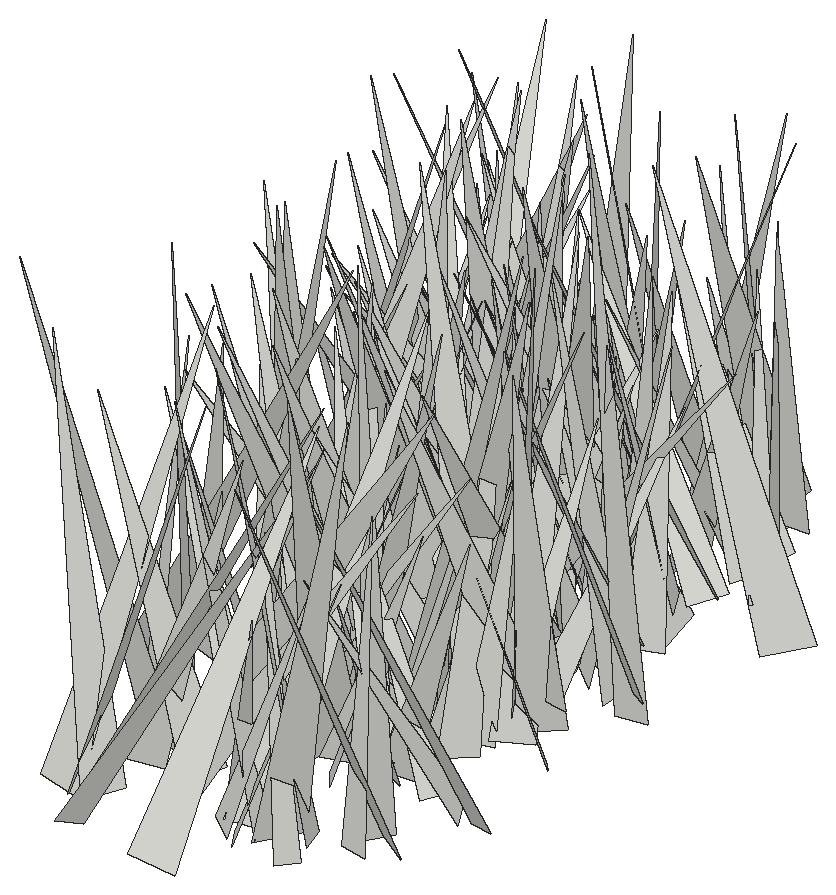
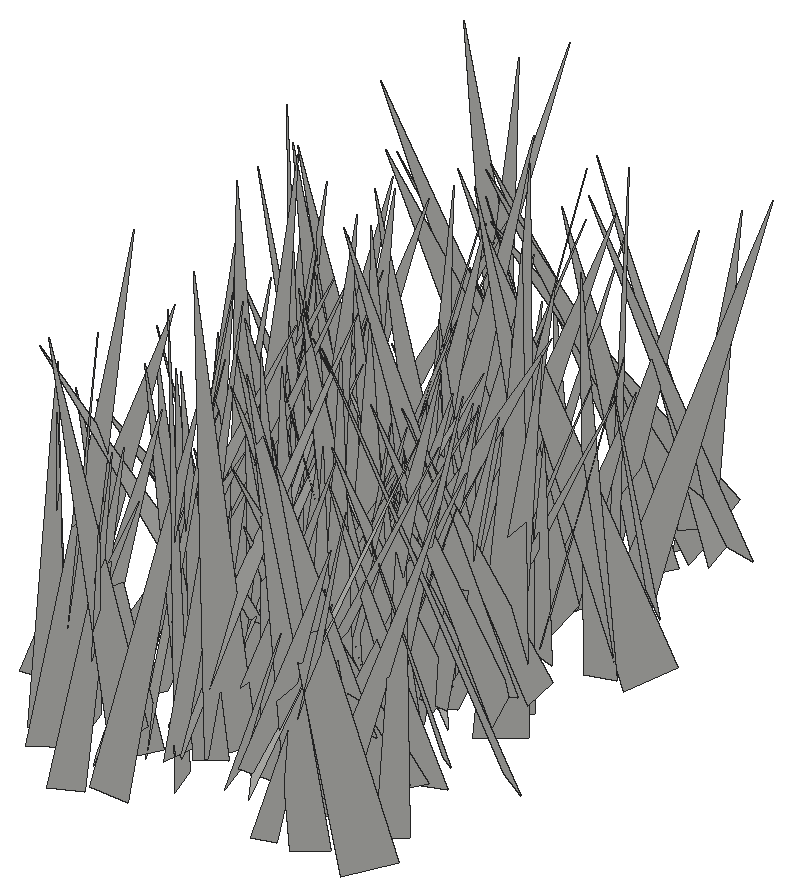
# SketchUp Ruby script. Lengths in inches.
U = 1.inch
M = Sketchup.active_model
def pt(a) = Geom::Point3d.new(a.map { |v| v * U })
def face(e, loops, mat)
  f = e.add_face(loops[0].map { |a| pt(a) })
  loops[1..].each { |l| e.add_face(l.map { |a| pt(a) }).erase! }
  f.material = f.back_material = mat if mat
  f
end
# faces: each face lists its corners as indices into pts; further lists are holes
def faces(e, pts, list, mat = nil) = list.each { |f| face(e, (f[0].is_a?(Array) ? f : [f]).map { |l| l.map { |i| pts[i] } }, mat) }
# xy, xz, yz: faces in a plane at the given z, y or x. An outline is a flat list of corners, or four numbers for a rectangle; further outlines are holes
def ring(l) = l.size == 4 ? [[l[0], l[1]], [l[2], l[1]], [l[2], l[3]], [l[0], l[3]]] : l.each_slice(2).to_a
def flat(e, list, mat, &to3) = list.each { |f| face(e, (f[0].is_a?(Array) ? f : [f]).map { |l| ring(l).map { |u, v| to3.(u, v) } }, mat) }
def xy(e, z, list, mat = nil) = flat(e, list, mat) { |x, y| [x, y, z] }
def xz(e, y, list, mat = nil) = flat(e, list, mat) { |x, z| [x, y, z] }
def yz(e, x, list, mat = nil) = flat(e, list, mat) { |y, z| [x, y, z] }
def lines(e, pts, list) = list.each { |a, b| e.add_line(pt(pts[a]), pt(pts[b])) }
# prism: a flat outline (further loops are holes) pulled along v
def prism(e, loops, v, mat = nil)
  f = face(e, loops, mat); d = Geom::Vector3d.new(v.map { |x| x * U })
  f.pushpull(f.normal.samedirection?(d) ? d.length : -d.length)
end
def box(e, o, s, mat = nil) = prism(e, [[o, [o[0] + s[0], o[1], o[2]], [o[0] + s[0], o[1] + s[1], o[2]], [o[0], o[1] + s[1], o[2]]]], [0, 0, s[2]], mat)
def at(x, y, z, deg = 0) = Geom::Transformation.translation(pt([x, y, z])) * Geom::Transformation.rotation(ORIGIN, Z_AXIS, deg.degrees)
def axes(o, x, y, z) = Geom::Transformation.new([*x, 0, *y, 0, *z, 0, *pt(o).to_a, 1])
def part(name) = M.definitions.add(name)
# library, detail: a bought-in or finely detailed component or shape, given as its bounding box
def library(name, o, s) = part(name).tap { |d| box(d.entities, o, s) }
def detail(e, o, s) = box(e.add_group.entities, o, s)
def put(e, d, t, mat = nil) = e.add_instance(d, t).tap { |i| i.material = mat if mat }
def group(e, t, mat = nil) = e.add_group.tap { |g| g.transformation = t; g.material = mat if mat }.entities
root = M.entities
c1 = part("fur_instance\#9")
p = [[0.8125,0,1.79],[0.67,-0.02,1.48],[0,-0.11,0],[0,0.11,0]]
faces(c1.entities,p,[[0,1,2,3]])
put(root,c1,axes([89.89,190.3,-27.1],[-4.18916,1.41328,1.44955],[1.84035,4.04661,1.3732],[0.84361,-1.80976,4.20247]))
put(root,c1,axes([88.07,187.8,-27.1],[2.28219,3.09258,0.57784],[3.14608,-2.24088,-0.43237],[0.01087,-0.72161,3.81909]))
put(root,c1,axes([86.96,186.11,-28.22],[4.54632,6.46757,0.61256],[6.48609,-4.47646,-0.87508],[0.36794,-1.0028,7.85702]))
put(root,c1,axes([91.4,174.74,-28.22],[-2.64388,-6.79077,2.11498],[-6.99476,2.07362,-2.08599],[-1.28885,2.67645,6.98236]))
put(root,c1,axes([87.72,190.74,-28.22],[5.48383,-1.63022,0.30334],[-1.45467,-5.23263,-1.82362],[-0.79597,-1.66854,5.42259]))
put(root,c1,axes([88.75,184.4,-27.1],[5.94248,2.0649,1.47313],[1.51819,-5.90154,2.14801],[-2.032,1.62942,5.91295]))
put(root,c1,axes([90.75,181.75,-27.1],[-5.69821,2.17721,0.97614],[2.15034,5.78116,-0.34192],[1.034,-0.02439,6.0904]))
put(root,c1,axes([90.47,175.18,-28.22],[2.37609,4.94692,0.8109],[4.47755,-2.49789,2.11838],[-2.25414,0.25283,5.06264]))
put(root,c1,axes([91.61,192.51,-27.1],[-5.39414,-3.77764,0.22745],[-3.78403,5.38986,-0.22257],[0.05845,0.31282,6.58162]))
put(root,c1,axes([90.58,188.05,-28.22],[-6.26748,-0.84521,1.62615],[-0.68504,6.45447,0.7145],[1.69984,-0.51518,6.28372]))
put(root,c1,axes([91.5625,190.9,-28.22],[-6.30755,-1.0303,0.95825],[-1.23667,6.15876,-1.51833],[0.67114,1.66527,6.20817]))
put(root,c1,axes([88.71,187.71,-28.22],[0.12132,5.40428,1.16344],[5.42728,0.10479,-1.05269],[1.05091,-1.16504,5.30215]))
put(root,c1,axes([89.95,191.67,-27.1],[4.40481,-2.70951,0.82389],[-1.71706,-3.76665,-3.20728],[-2.2521,-2.42766,4.05674]))
put(root,c1,axes([90.42,189.11,-27.1],[-4.33285,5.33033,0.39838],[5.19442,4.31986,-1.30443],[1.26061,0.52067,6.74422]))
put(root,c1,axes([89.58,190.12,-28.22],[1.06055,3.50039,1.15885],[3.68372,-1.05849,-0.17402],[-0.16095,-1.16074,3.65339]))
put(root,c1,axes([88.96,184.14,-28.22],[5.45655,-4.97036,1.37233],[-4.9464,-5.60993,-0.6508],[-1.45634,0.43117,7.35221]))
put(root,c1,axes([91.19,179.65,-28.22],[-0.14147,5.00237,0.6936],[4.87308,-0.04695,1.33257],[-1.32587,-0.70632,4.82369]))
put(root,c1,axes([91.25,183.76,-28.22],[-5.28354,-0.86585,0.73138],[-0.45173,4.80676,2.42722],[1.0395,-2.31209,4.77222]))
put(root,c1,axes([91.92,187.52,-28.22],[-1.59145,-6.67923,2.98055],[-7.18236,0.85085,-1.92829],[-1.38185,3.26993,6.58988]))
put(root,c1,axes([88.44,182.95,-27.1],[5.14686,-0.10254,0.48257],[-0.21946,-5.00543,1.27711],[-0.44184,1.29176,4.98695]))
put(root,c1,axes([88.93,179.57,-28.22],[-0.17668,-5.97479,1.5156],[-5.97573,0.53792,1.42395],[1.51188,1.4279,5.80532]))
put(root,c1,axes([92.4,190,-27.1],[-5.87087,-0.65311,0.1721],[-0.62527,5.82501,0.77566],[0.25536,-0.75237,5.85594]))
put(root,c1,axes([91.77,171.64,-28.22],[-6.40273,2.01611,1.14645],[1.98655,6.50456,-0.34415],[1.19695,-0.01086,6.70383]))
put(root,c1,axes([90.48,185.39,-27.1],[-0.08561,-4.51883,0.61864],[-4.55746,0.06047,-0.18896],[-0.17898,0.62161,4.51569]))
put(root,c1,axes([90.54,193.22,-28.22],[2.63547,-2.52355,0.88422],[-2.24578,-2.7628,-1.19134],[-1.45143,-0.30736,3.44888]))
put(root,c1,axes([91.93,191.88,-27.1],[-2.38269,3.95567,1.05235],[4.03891,2.07425,1.34786],[-0.66484,-1.57548,4.41677]))
put(root,c1,axes([92.6875,180.37,-28.22],[-5.83458,-0.97839,0.23219],[-1.00024,5.78729,-0.74851],[0.10327,0.77686,5.8685]))
put(root,c1,axes([87.0625,192.63,-28.22],[4.73655,-6.32836,0.37656],[-6.13582,-4.45802,2.25891],[1.59428,1.644,7.57499]))
put(root,c1,axes([90.7,176.82,-28.22],[-4.49865,-5.44108,2.87885],[-5.83326,4.90701,0.15896],[1.96626,2.10876,7.05818]))
put(root,c1,axes([92.63,176.8125,-28.22],[-2.13288,4.47426,0.69403],[4.36785,1.83113,1.61826],[-1.19274,-1.2953,4.68502]))
put(root,c1,axes([89.04,183.8125,-27.1],[4.0967,-0.1052,0.02727],[-0.10864,-3.93802,1.12914],[0.00278,1.12946,3.93942]))
put(root,c1,axes([89.52,183.01,-28.22],[7.83218,-2.47016,1.5817],[-2.12062,-7.88445,-1.81244],[-2.02643,-1.29626,8.00998]))
put(root,c1,axes([90.46,182.61,-27.1],[1.50954,-3.07856,1.78204],[-3.55315,-1.39659,0.59714],[-0.16832,1.87187,3.37633]))
put(root,c1,axes([91.59,178.93,-28.22],[-3.92886,-2.51502,0.86647],[-2.44083,4.02285,0.60923],[1.05758,-0.05874,4.62495]))
put(root,c1,axes([91.67,185.23,-28.22],[3.58153,-3.37168,2.12142],[-3.21603,-4.13077,-1.13573],[-2.3507,0.51427,4.78599]))
put(root,c1,axes([92.67,184.25,-27.1],[-3.84784,-1.19504,0.32807],[-1.23606,3.62421,-1.29571],[-0.08892,1.33363,3.81512]))
put(root,c1,axes([90.45,185,-27.1],[4.99403,0.89918,1.35491],[0.3935,-4.91429,1.81096],[-1.5778,1.62046,4.74018]))
put(root,c1,axes([91.96,186.64,-27.1],[-3.17916,-2.57933,0.00353],[-2.53731,3.12837,0.73174],[0.46373,-0.56605,4.02798]))
put(root,c1,axes([89.2,188.12,-28.22],[-0.99691,5.86129,1.26655],[5.41282,1.43213,-2.36709],[2.58075,-0.73958,5.45394]))
put(root,c1,axes([91.16,191.28,-28.22],[5.03177,-2.92165,1.14225],[-2.20313,-4.82824,-2.64459],[-2.23316,-1.81978,5.18275]))
put(root,c1,axes([89.12,192.84,-28.22],[0.83878,-6.84447,1.51714],[-6.71971,-0.34936,2.13903],[1.99848,1.69801,6.55552]))
put(root,c1,axes([89.86,190.82,-28.22],[6.15158,-3.29467,0.71793],[-3.15743,-6.15236,-1.17953],[-1.18361,-0.7112,6.87789]))
put(root,c1,axes([90.54,171.24,-28.22],[1.55056,7.17303,0.47228],[7.18686,-1.53634,-0.26142],[0.15632,-0.51668,7.33405]))
put(root,c1,axes([87.71,178.71,-28.22],[7.56022,-3.29271,0.03526],[-3.23696,-7.41517,1.59297],[0.60437,1.47429,8.09082]))
put(root,c1,axes([92,188.82,-27.1],[-5.13165,1.21269,1.54361],[1.09048,5.35359,-0.58061],[1.63224,0.23592,5.24093]))
put(root,c1,axes([93.08,190.19,-28.22],[-6.30471,-1.37126,0.42808],[-1.05468,5.72683,2.8114],[0.97532,-2.67133,5.80738]))
put(root,c1,axes([89.42,183.91,-27.1],[0.24663,7.62872,2.41582],[7.70784,0.42293,-2.12242],[2.15005,-2.39126,7.33168]))
put(root,c1,axes([93.79,186.91,-28.22],[-0.45254,-7.13046,0.09555],[-6.72101,0.39447,-2.39372],[-2.38342,0.24148,6.7319]))
put(root,c1,axes([89.21,188.96,-28.22],[6.84085,-1.05323,0.60817],[-1.14548,-6.7472,1.19982],[-0.40871,1.28156,6.81667]))
put(root,c1,axes([93.53,190.91,-28.22],[-4.16837,-0.36819,0.02902],[-0.35612,3.91965,-1.4217],[-0.09791,1.41863,3.93569]))
put(root,c1,axes([92.87,181.38,-28.22],[-3.95377,2.90545,0.68572],[2.92437,3.99824,-0.07937],[0.59996,-0.34142,4.90588]))
put(root,c1,axes([93.03,179.86,-28.22],[-4.7653,3.97573,1.88545],[4.327,4.73874,0.94381],[0.79899,-1.95123,6.13381]))
put(root,c1,axes([93.35,174.18,-28.22],[-5.50696,2.25656,1.40845],[2.52369,5.45565,1.12666],[0.84072,-1.59571,5.84374]))
put(root,c1,axes([93.37,184.85,-27.1],[0.69074,-4.72184,2.34998],[-4.89788,-1.45354,-1.48096],[-1.95676,1.97148,4.53648]))
put(root,c1,axes([91.79,177.77,-28.22],[-7.4216,0.05563,3.73189],[-0.80703,8.0859,-1.72548],[3.64401,1.90407,7.21845]))
put(root,c1,axes([93.91,185.04,-28.22],[-6.19983,-0.76734,1.02255],[-1.02443,6.01091,-1.70052],[0.76483,1.83095,6.01123]))
put(root,c1,axes([93.95,190.33,-27.1],[-5.48132,1.03762,0.48302],[1.07413,5.47965,0.41785],[0.39525,-0.50168,5.563]))
put(root,c1,axes([91.5,182.15,-28.22],[5.47744,-1.647,1.93505],[-1.81976,-5.75174,0.25556],[-1.77356,0.81501,5.71398]))
put(root,c1,axes([91.14,187.47,-27.1],[5.12672,-4.5376,2.59386],[-5.0883,-5.16347,1.02416],[-1.19461,2.5199,6.76936]))
put(root,c1,axes([90.95,184.17,-28.22],[4.55508,3.875,0.43107],[3.83788,-4.57312,0.55448],[-0.68713,0.14532,5.95457]))
put(root,c1,axes([93.59,180.89,-28.22],[0.79588,-7.21699,0.96951],[-7.03929,-1.01213,-1.75565],[-1.86367,0.74092,7.04528]))
put(root,c1,axes([94.33,184.31,-27.1],[-2.33068,3.85921,0.35584],[3.66264,2.05758,1.6744],[-1.26695,-1.15111,4.18592]))
put(root,c1,axes([93.42,184.85,-28.22],[-3.76745,6.43232,1.47995],[6.58457,3.78058,0.33053],[0.45645,-1.44608,7.44709]))
put(root,c1,axes([92.72,182.76,-28.22],[4.14575,-5.15062,1.64406],[-4.88287,-4.45639,-1.64839],[-2.32151,0.17524,6.40304]))
put(root,c1,axes([90.77,171.76,-28.22],[6.34041,1.92452,0.88463],[1.94009,-6.39712,0.01179],[-0.84995,-0.24555,6.62604]))
put(root,c1,axes([92.32,185.88,-28.22],[1.9178,-7.47283,0.23219],[-7.45531,-1.92947,-0.52008],[-0.56157,0.09505,7.69744]))
put(root,c1,axes([94.78,188.15,-27.1],[-2.52034,-4.28654,0.32351],[-4.12689,2.30776,-1.57296],[-1.20326,1.06349,4.71724]))
put(root,c1,axes([94.93,185.02,-27.1],[-3.76268,-4.24685,0.11424],[-4.17448,3.66755,-1.15295],[-0.78896,0.84846,5.55555]))
put(root,c1,axes([94.97,191.81,-27.1],[-4.99858,-6.00178,0.67378],[-6.03784,4.94565,-0.739],[-0.1407,0.9901,7.77567]))
put(root,c1,axes([93.3,187.06,-28.22],[-6.63675,3.07759,1.929],[2.57186,6.8191,-2.03087],[2.56478,1.12578,7.02806]))
put(root,c1,axes([90.63,186.8125,-28.22],[3.49272,-6.19271,0.17705],[-6.11252,-3.41157,1.25629],[1.00898,0.76914,6.99789]))
put(root,c1,axes([92.36,181.63,-28.22],[2.6007,2.51832,0.88377],[2.64819,-2.58836,-0.41733],[-0.33183,-0.9193,3.59603]))
put(root,c1,axes([94.68,179.875,-28.22],[0.07199,5.81915,0.58708],[5.58747,-0.24194,1.7129],[-1.72841,-0.53974,5.5618]))
put(root,c1,axes([94.32,182.6875,-27.1],[-3.93279,-0.23592,0.50656],[-0.05149,3.7386,1.34138],[0.55643,-1.32147,3.70448]))
put(root,c1,axes([91.81,182.15,-27.1],[4.67763,2.46387,0.32375],[2.42875,-4.67875,0.51598],[-0.52599,0.30722,5.26162]))
put(root,c1,axes([91.51,173.67,-28.22],[3.48254,-4.50934,1.30252],[-4.66936,-3.1635,1.53235],[0.47726,1.95368,5.48763]))
put(root,c1,axes([93.95,185.22,-27.1],[-5.87667,-3.9224,1.1719],[-3.54254,5.90008,1.98324],[2.05159,-1.04767,6.78139]))
put(root,c1,axes([93.13,188,-27.1],[2.46891,-7.20313,1.70316],[-7.36136,-2.57683,-0.22704],[-0.77207,1.53499,7.61111]))
put(root,c1,axes([94.59,186.66,-28.22],[-6.34287,-0.8603,1.40577],[-0.30586,6.10717,2.3574],[1.61949,-2.21602,5.95103]))
put(root,c1,axes([95.03,180.51,-28.22],[-6.61379,-2.13915,0.88077],[-1.88588,6.53057,1.69974],[1.33985,-1.36736,6.74011]))
put(root,c1,axes([93.04,184.2,-27.1],[-5.61419,2.77509,3.47904],[3.15086,6.4338,-0.04739],[3.14276,-1.49299,6.26243]))
put(root,c1,axes([92.8,185.67,-27.1],[3.62084,3.81527,1.03017],[3.87963,-3.69771,0.05854],[-0.75237,-0.70613,5.25959]))
put(root,c1,axes([92.43,189.99,-27.1],[2.19919,-5.46865,1.19281],[-5.58851,-2.07385,0.79564],[0.31218,1.39943,5.84033]))
put(root,c1,axes([93.65,188.26,-28.22],[5.0258,-2.8928,2.35137],[-3.11716,-5.42578,-0.01254],[-2.04464,1.16127,5.79886]))
put(root,c1,axes([94.42,185.65,-28.22],[-4.05374,2.9207,0.15477],[2.65047,3.78022,-1.91631],[1.23673,1.47198,4.61422]))
put(root,c1,axes([95.3,183.08,-27.1],[-7.34828,2.49323,1.09592],[2.03506,7.1224,-2.5582],[1.80991,2.11416,7.32591]))
put(root,c1,axes([91.37,171.7,-28.22],[7.04502,0.38941,0.11832],[0.34745,-6.82295,1.76766],[-0.21195,1.75889,6.83077]))
put(root,c1,axes([93.3125,191.28,-27.1],[6.93717,-2.75986,2.51351],[-2.97128,-7.29338,0.19237],[-2.25967,1.11744,7.46352]))
put(root,c1,axes([93.72,191.68,-27.1],[-0.85908,-3.57953,0.71794],[-3.54097,0.99653,0.73143],[0.88884,0.51028,3.60778]))
put(root,c1,axes([93.08,186.85,-28.22],[3.19088,3.17646,1.19509],[3.39239,-3.03309,-0.99593],[-0.09903,-1.55252,4.39087]))
put(root,c1,axes([92.04,169.82,-28.22],[6.45135,0.1489,0.38361],[-0.04006,-5.77049,2.9136],[-0.40954,2.91007,5.75787]))
put(root,c1,axes([93.34,184.78,-27.1],[3.78435,-1.32179,0.68035],[-1.35222,-3.83372,0.07338],[-0.61764,0.29457,4.00787]))
put(root,c1,axes([91.74,175.77,-28.22],[5.30447,3.34271,0.68413],[3.37643,-4.96043,-1.94241],[0.49141,-1.99988,5.96139]))
put(root,c1,axes([94.43,192.38,-27.1],[6.50516,0.09741,3.11354],[0.81371,-7.01185,-1.48071],[-3.00691,-1.68675,6.33514]))
put(root,c1,axes([95.31,178.63,-28.22],[-4.4668,1.24969,0.75909],[0.98308,4.37301,-1.41442],[1.08236,1.18546,4.4174]))
put(root,c1,axes([96.67,172.69,-28.22],[-6.17227,-0.98801,0.5453],[-1.07692,6.06305,-1.2042],[0.3373,1.27815,6.13375]))
put(root,c1,axes([92.95,185.06,-28.22],[1.22352,3.80068,0.33063],[3.61313,-1.04295,-1.38167],[1.22465,-0.72012,3.74608]))
put(root,c1,axes([96.34,188.91,-28.22],[-3.64802,-5.0358,0.07825],[-5.03596,3.64854,0.02575],[0.06676,0.04827,6.21825]))
put(root,c1,axes([94.91,180.98,-28.22],[6.13444,-4.45258,1.42838],[-3.84619,-6.14459,-2.6359],[-2.65943,-1.38408,7.10696]))
put(root,c1,axes([96.61,178.06,-28.22],[-3.18645,2.79123,0.05753],[2.78151,3.16651,0.42911],[-0.23972,-0.36053,4.21429]))
put(root,c1,axes([95.81,185.05,-28.22],[2.37526,2.53476,1.46683],[2.25858,-2.78775,1.16004],[-1.86424,-0.14786,3.27432]))
put(root,c1,axes([93.49,192,-27.1],[0.81031,-5.69395,0.84212],[-5.55553,-0.55126,1.61834],[1.50543,1.03047,5.51893]))
put(root,c1,axes([96.8125,185.18,-28.22],[-5.93651,2.05948,0.4431],[1.83167,5.70073,-1.95618],[1.04056,1.71471,5.97135]))
put(root,c1,axes([94.57,191.99,-28.22],[6.58164,2.52237,2.667],[2.99732,-6.85363,-0.91486],[-2.11926,-1.85972,6.9888]))
put(root,c1,axes([96.6,182.25,-27.1],[5.34271,-3.44394,4.19103],[-3.85612,-6.54857,-0.46545],[-3.8152,1.796,6.33945]))
put(root,c1,axes([96.9375,190.79,-28.22],[-5.96506,-5.04673,2.13711],[-5.35643,6.03696,-0.69462],[1.15994,1.92465,7.7826]))
put(root,c1,axes([96.31,180.875,-28.22],[-4.83197,-1.5354,1.95575],[-2.0901,4.8234,-1.3772],[1.34681,1.9768,4.87942]))
put(root,c1,axes([94.17,186.7,-28.22],[0.05703,4.78722,0.58826],[4.57544,0.13244,-1.52137],[1.52606,-0.57598,4.5394]))
put(root,c1,axes([95.77,193.91,-28.22],[0.0355,-6.28923,0.69696],[-6.32457,-0.05728,-0.19472],[-0.19984,0.69551,6.28631]))
put(root,c1,axes([92.51,179.2,-28.22],[4.14208,3.82367,0.06036],[3.46383,-3.71363,-2.44781],[1.62049,-1.8356,5.07794]))
put(root,c1,axes([94.65,174.04,-28.22],[3.65052,-1.24636,0.3015],[-1.17659,-3.61738,-0.70767],[-0.50984,-0.576,3.79195]))
put(root,c1,axes([96.55,187.38,-28.22],[-4.07639,-4.57708,0.71562],[-4.52519,4.13816,0.69067],[0.99219,0.06853,6.09012]))
put(root,c1,axes([97.87,173.24,-28.22],[-6.23091,-2.8217,1.23434],[-3.03851,6.08694,-1.42355],[0.50305,1.81577,6.69027]))
put(root,c1,axes([97.27,185.95,-28.22],[-6.52757,-2.25287,1.08541],[-2.07972,6.57544,1.14066],[1.38863,-0.74224,6.81054]))
put(root,c1,axes([94.46,179.59,-28.22],[6.6153,-1.38256,1.33275],[-1.44359,-6.733,0.18083],[-1.26639,0.45296,6.75581]))
put(root,c1,axes([95.28,169.38,-28.22],[-1.05391,6.67902,0.37292],[6.52998,1.10912,-1.41007],[1.4518,-0.14015,6.613]))
put(root,c1,axes([95.07,188.61,-27.1],[7.37439,-3.31849,1.28024],[-2.90244,-7.31769,-2.24953],[-2.05603,-1.57231,7.76747]))
put(root,c1,axes([96.77,186.625,-28.22],[-3.85021,0.78609,0.9669],[0.45373,3.80886,-1.28983],[1.16059,1.11875,3.71193]))
put(root,c1,axes([94.95,190.9,-27.1],[5.5976,-0.64404,1.05715],[-0.59203,-5.69245,-0.3332],[-1.08713,-0.21617,5.62467]))
put(root,c1,axes([99.21,188.96,-27.1],[-3.06534,4.86368,0.18481],[4.51167,2.75744,2.26433],[-1.82603,-1.35165,5.28436]))
put(root,c1,axes([91.85,176.3125,-28.22],[3.5795,-7.50714,1.0436],[-6.77337,-2.6505,4.166],[3.40115,2.62237,7.19823]))
put(root,c1,axes([98.49,188.5,-28.22],[-7.42366,-0.80204,0.92134],[-0.52005,7.2098,2.08597],[1.1053,-1.9946,7.16957]))
put(root,c1,axes([97.33,182.35,-28.22],[-5.53054,0.45224,1.5037],[0.10523,5.59989,-1.29715],[1.5667,1.22031,5.39525]))
put(root,c1,axes([95.2,177.51,-28.22],[6.57894,-4.30915,0.69378],[-4.10201,-6.53322,-1.6802],[-1.49116,-1.03963,7.68298]))
put(root,c1,axes([98.1875,171.72,-28.22],[-4.58917,0.765,0.19448],[0.68534,4.43094,-1.25723],[0.3916,1.21042,4.47941]))
put(root,c1,axes([94.2,189,-28.22],[2.66865,-7.95792,0.14871],[-7.80747,-2.5868,1.68053],[1.54726,0.67254,8.22351]))
put(root,c1,axes([97.03,185.32,-27.1],[-4.89402,-3.33819,1.83703],[-3.30827,5.20635,0.64726],[1.89038,0.46913,5.88863]))
put(root,c1,axes([98.95,189.36,-27.1],[-3.68425,-5.36529,0.32526],[-5.32374,3.58793,-1.11818],[-0.74155,0.8979,6.41168]))
put(root,c1,axes([95.48,172.2,-28.22],[2.51167,3.62255,0.80621],[3.69421,-2.34748,-0.96099],[0.35452,-1.20325,4.30208]))
put(root,c1,axes([97.32,192.625,-28.22],[-4.40501,-3.46188,0.56585],[-3.18391,4.32713,1.68747],[1.47225,-1.00011,5.34239]))
put(root,c1,axes([93.16,173.82,-28.22],[4.41498,5.25807,0.18984],[4.81628,-3.93899,-2.90917],[2.11822,-2.00311,6.21901]))
put(root,c1,axes([97.64,185.59,-28.22],[-3.80527,0.70423,0.62745],[0.3357,3.44844,-1.83447],[0.88144,1.72686,3.40746]))
put(root,c1,axes([96.03,186.33,-27.1],[3.36091,-1.13304,0.9234],[-1.35023,-3.29337,0.87337],[-0.55977,1.1411,3.43755]))
put(root,c1,axes([96.17,172.76,-28.22],[-4.73234,6.09922,1.47861],[5.53404,4.92888,-2.61961],[2.95993,0.53615,7.26177]))
put(root,c1,axes([95.5625,177.14,-28.22],[3.11489,-2.67244,0.85057],[-2.80172,-2.90834,1.1224],[0.12545,1.40269,3.94774]))
put(root,c1,axes([99.24,174.47,-28.22],[-7.91635,-0.39433,1.24518],[-0.80795,7.48837,-2.76517],[1.02625,2.85367,7.42819]))
put(root,c1,axes([97.52,192.41,-27.1],[-3.69275,-0.52533,1.17947],[-0.76187,3.77166,-0.70545],[1.04243,0.89562,3.66261]))
put(root,c1,axes([96.125,176.17,-28.22],[3.13129,2.44329,0.37399],[2.42945,-3.15346,0.26073],[-0.45532,-0.0231,3.96316]))
put(root,c1,axes([95.13,181.51,-28.22],[6.3266,0.04535,0.7535],[-0.10627,-6.24313,1.26797],[-0.74735,1.27161,6.1984]))
put(root,c1,axes([96.28,182.79,-27.1],[3.51282,6.48869,2.15536],[6.79895,-3.57131,-0.32959],[-0.72316,-2.057,7.37118]))
put(root,c1,axes([97.03,177.46,-28.22],[3.44077,4.42208,0.21812],[4.18127,-3.33634,1.68138],[-1.45578,0.8691,5.34478]))
put(root,c1,axes([98.62,191.36,-27.1],[-5.41908,-0.82486,1.13145],[-1.12996,5.24719,-1.58656],[0.82691,1.76453,5.24687]))
put(root,c1,axes([96.93,194.45,-28.22],[3.85472,-3.45884,0.89823],[-3.26491,-3.94586,-1.18314],[-1.45282,-0.30973,5.04209]))
put(root,c1,axes([96.15,171.9,-28.22],[3.52648,2.43175,0.31475],[2.41999,-3.54045,0.23962],[-0.3951,0.0194,4.27692]))
put(root,c1,axes([95.77,180.27,-28.22],[7.6269,-0.50277,1.8471],[-0.68475,-7.80192,0.70374],[-1.78765,0.84341,7.61099]))
put(root,c1,axes([96.76,188.82,-27.1],[0.02782,-4.7345,1.86898],[-5.06027,0.17616,0.52158],[0.54982,1.86087,4.70577]))
put(root,c1,axes([96.21,192.43,-27.1],[6.43486,-0.85229,1.84553],[-1.08084,-6.62327,0.70985],[-1.72168,0.97247,6.45212]))
put(root,c1,axes([97.99,186.4,-27.1],[1.8485,-3.49978,1.33816],[-3.45042,-2.17169,-0.91344],[-1.46071,0.70098,3.8511]))
put(root,c1,axes([97.41,177.29,-28.22],[-1.12897,-3.54048,0.33773],[-3.515,1.16474,0.46018],[0.54205,0.17891,3.68752]))
put(root,c1,axes([95.18,182.75,-28.22],[6.15872,-4.73604,0.69713],[-4.78091,-6.14284,0.50431],[-0.2428,0.82545,7.75278]))
put(root,c1,axes([98.75,180.91,-28.22],[-6.53703,2.92768,0.70077],[2.53956,6.26275,-2.47462],[1.61648,2.00045,6.72163]))
put(root,c1,axes([99.01,177.24,-28.22],[-3.1283,2.85302,0.75954],[2.94685,2.94951,1.058],[-0.18092,-1.28978,4.09959]))
put(root,c1,axes([97.07,179.52,-28.22],[2.13777,3.57515,0.4757],[3.58502,-2.16686,0.17428],[-0.39447,-0.3179,4.1619]))
put(root,c1,axes([98.11,179.33,-28.22],[-5.56085,2.56326,1.5764],[2.25423,5.74256,-1.38556],[1.99343,0.65656,5.96435]))
put(root,c1,axes([98.54,181.68,-27.1],[2.87814,-5.28951,1.31735],[-4.95416,-3.15966,-1.86304],[-2.27391,0.18887,5.72641]))
put(root,c1,axes([99.34,191.99,-27.1],[-3.99444,1.28958,0.25526],[1.31279,3.95594,0.55757],[0.06915,-0.60932,4.16025]))
put(root,c1,axes([97.1,184.0625,-27.1],[5.11337,-4.37567,0.02712],[-4.08728,-4.79107,-2.37351],[-1.56248,-1.78687,6.29758]))
put(root,c1,axes([99.27,190.67,-27.1],[-4.79619,2.23097,0.90337],[2.34699,4.78153,0.65218],[0.53379,-0.97799,5.24932]))
put(root,c1,axes([100.39,180.41,-28.22],[-3.99392,-3.16377,0.39905],[-3.06383,3.62986,-1.88605],[-0.88412,1.71311,4.73326]))
put(root,c1,axes([95.3125,185.39,-27.1],[4.61387,-2.10989,0.31356],[-1.93342,-3.82099,2.73855],[0.90102,2.60502,4.2708]))
put(root,c1,axes([98.65,188.24,-27.1],[-4.19066,-2.50752,1.09961],[-2.47633,4.32875,0.43379],[1.16817,0.18082,4.86427]))
put(root,c1,axes([97.38,187.27,-27.1],[2.10827,-4.41232,0.88185],[-4.4927,-2.11805,0.1432],[-0.24874,0.85808,4.88803]))
put(root,c1,axes([98.84,192.19,-27.1],[-5.61783,-2.93903,2.21928],[-3.25584,5.85535,-0.48739],[1.72124,1.48327,6.32142]))
put(root,c1,axes([97.5,185.3125,-28.22],[6.81061,4.1437,0.72104],[3.52808,-6.3754,3.31382],[-2.28972,2.50169,7.25074]))
put(root,c1,axes([98.98,185.91,-27.1],[-1.13114,-4.608,0.05517],[-4.59723,1.12439,-0.34274],[-0.31976,0.13515,4.73241]))
put(root,c1,axes([99.39,184.83,-28.22],[-6.3571,-0.05635,1.63328],[-0.03082,6.56286,0.10646],[1.63396,-0.09544,6.35645]))
put(root,c1,axes([96.46,191.41,-28.22],[4.6953,-3.04636,0.27903],[-3.0591,-4.67738,0.40996],[-0.01004,0.49581,5.58194]))
put(root,c1,axes([97.65,194.33,-27.1],[7.10031,-2.91459,1.55919],[-2.29482,-7.00551,-2.64516],[-2.37902,-1.94118,7.20502]))
put(root,c1,axes([98.33,187.2,-28.22],[-2.20726,4.7722,2.01563],[5.04733,2.47451,-0.33147],[1.16667,-1.67676,5.24748]))
put(root,c1,axes([98.29,181.24,-28.22],[-2.91269,3.59929,0.76549],[3.33369,2.99435,-1.39463],[1.55801,0.3218,4.41516]))
put(root,c1,axes([100.52,183.94,-28.22],[1.70019,7.5386,2.42367],[7.33263,-2.43467,2.42902],[-2.9895,-1.68439,7.33628]))
put(root,c1,axes([98.03,180.27,-28.22],[-1.6675,3.7386,1.84502],[3.94069,2.06209,-0.61692],[1.36097,-1.39013,4.04687]))
put(root,c1,axes([98.22,182.79,-28.22],[-3.43381,3.18637,0.41007],[2.54254,3.06224,-2.50406],[1.96382,1.60682,3.959]))
put(root,c1,axes([99.45,181.74,-27.1],[1.25077,5.74635,3.18749],[6.40163,-1.79789,0.7292],[-1.48314,-2.91412,5.83551]))
put(root,c1,axes([97.07,172.76,-28.22],[6.75458,-3.1446,1.55563],[-3.25939,-6.87331,0.25842],[-1.29802,0.89549,7.44621]))
put(root,c1,axes([101.18,183.43,-27.1],[-4.07281,-4.5818,0.7427],[-4.55178,3.7491,-1.83244],[-0.90871,1.75604,5.85003]))
put(root,c1,axes([101.11,176.6,-28.22],[-2.79932,-5.24784,0.26282],[-5.09915,2.64134,-1.57068],[-1.26789,0.96362,5.73663]))
put(root,c1,axes([99.18,173.39,-28.22],[1.36793,4.62634,1.5435],[4.80198,-1.5578,0.41343],[-0.85231,-1.35162,4.8066]))
put(root,c1,axes([98.06,182.08,-28.22],[7.03768,2.72348,2.80411],[3.28727,-7.24831,-1.21043],[-2.11523,-2.20318,7.44856]))
put(root,c1,axes([100.06,177.04,-28.22],[-4.30266,-2.43803,0.04686],[-2.30354,4.09498,1.544],[0.79994,-1.32144,4.69819]))
put(root,c1,axes([97.9375,185.05,-28.22],[3.37327,4.28522,1.21914],[4.44713,-3.33099,-0.5966],[-0.2692,-1.33033,5.4209]))
put(root,c1,axes([98.36,193.58,-27.1],[1.13187,-5.42392,1.09616],[-5.52646,-1.05128,0.50466],[0.2806,1.17367,5.51773]))
put(root,c1,axes([99.65,174.38,-28.22],[-3.38776,-6.42257,0.32475],[-6.36234,3.40084,0.88702],[0.93573,-0.12917,7.20691]))
put(root,c1,axes([100.59,189.67,-27.1],[-4.5545,1.12209,0.15618],[1.0267,4.36161,-1.39615],[0.47894,1.3207,4.4781]))
put(root,c1,axes([97.43,177.49,-28.22],[2.4486,-4.30122,0.69777],[-4.269,-2.2075,1.37318],[0.8735,1.26866,4.75506]))
put(root,c1,axes([101.47,189.67,-28.22],[-4.16416,5.80884,2.0419],[6.1268,3.66414,2.07088],[-0.6118,-2.84317,6.84063]))
put(root,c1,axes([100.1875,190.6,-27.1],[-4.76219,-1.42096,1.84075],[-1.91994,4.76946,-1.2853],[1.31199,1.82182,4.80058]))
put(root,c1,axes([98.98,181.93,-28.22],[3.86717,-5.0611,1.49434],[-5.13106,-4.03908,-0.40116],[-1.23289,0.93486,6.35679]))
